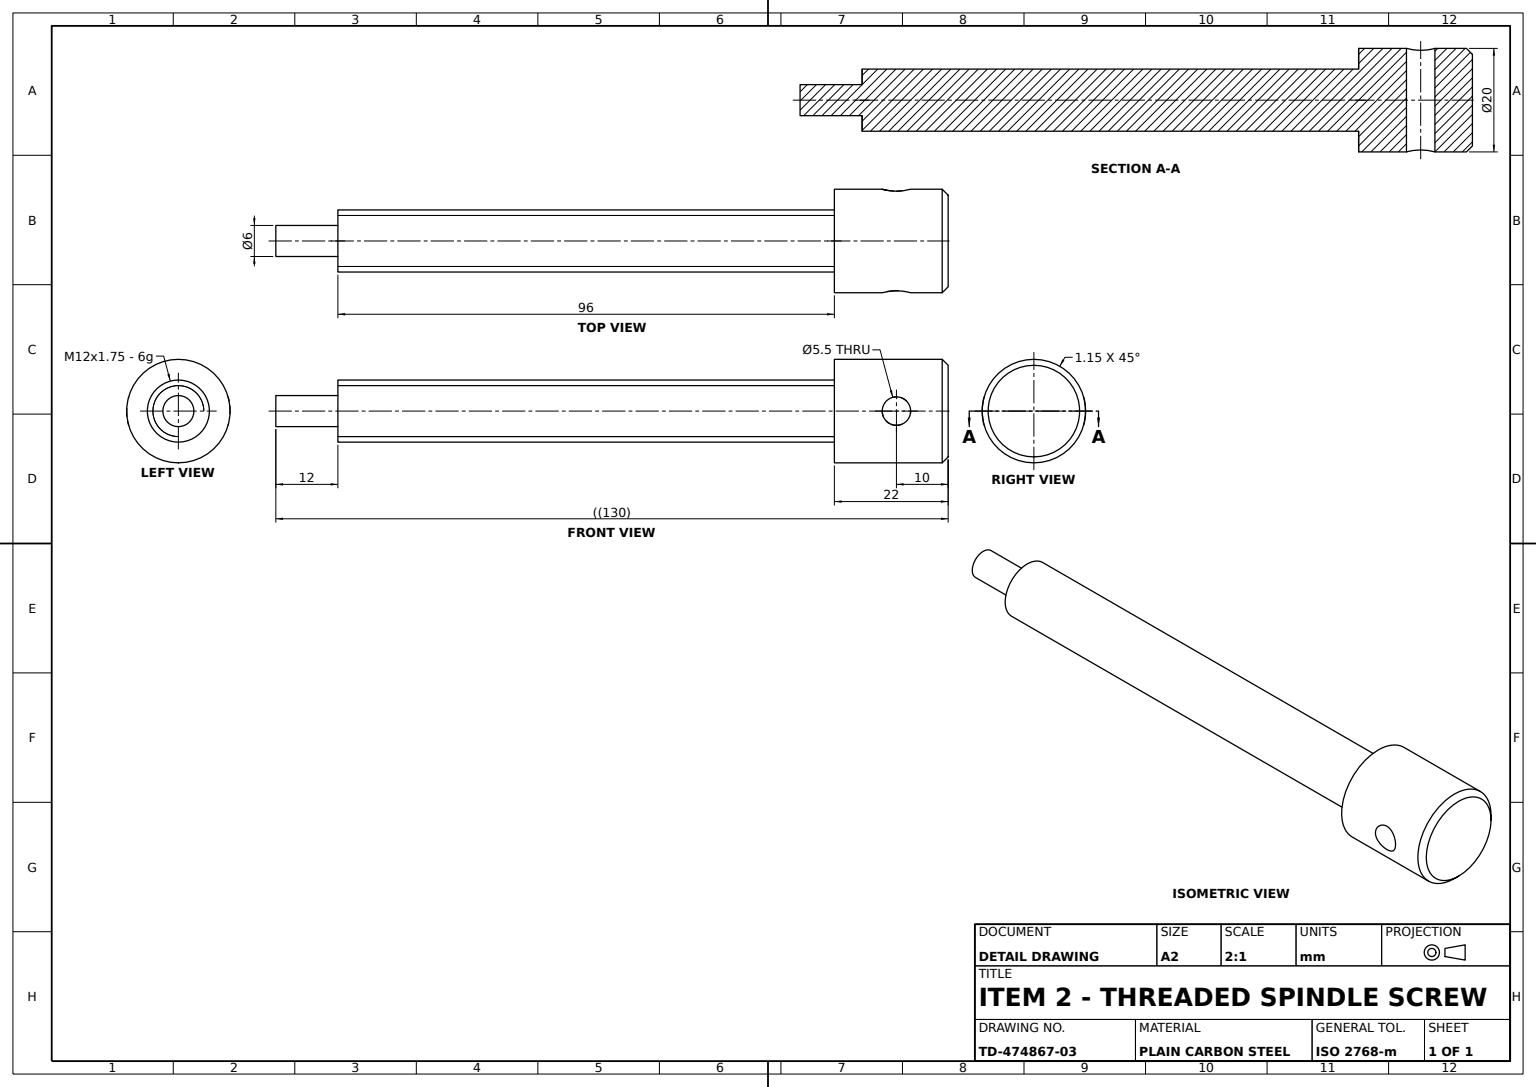
ISO-10303-21;
HEADER;
FILE_DESCRIPTION((''),'2;1');
FILE_NAME('','',(''),(''),'','','');
FILE_SCHEMA(('AUTOMOTIVE_DESIGN'));
ENDSEC;
DATA;
#1=APPLICATION_CONTEXT('');
#2=PRODUCT_CONTEXT('',#1,'mechanical');
#3=PRODUCT('','','',(#2));
#4=PRODUCT_DEFINITION_FORMATION('','',#3);
#5=PRODUCT_DEFINITION_CONTEXT('',#1,'design');
#6=PRODUCT_DEFINITION('','',#4,#5);
#7=PRODUCT_DEFINITION_SHAPE('','',#6);
#8=(LENGTH_UNIT()NAMED_UNIT(*)SI_UNIT(.MILLI.,.METRE.));
#9=(NAMED_UNIT(*)PLANE_ANGLE_UNIT()SI_UNIT($,.RADIAN.));
#10=(NAMED_UNIT(*)SI_UNIT($,.STERADIAN.)SOLID_ANGLE_UNIT());
#11=UNCERTAINTY_MEASURE_WITH_UNIT(LENGTH_MEASURE(1.E-05),#8,'distance_accuracy_value','');
#12=(GEOMETRIC_REPRESENTATION_CONTEXT(3)GLOBAL_UNCERTAINTY_ASSIGNED_CONTEXT((#11))GLOBAL_UNIT_ASSIGNED_CONTEXT((#8,#9,#10))REPRESENTATION_CONTEXT('',''));
#13=CARTESIAN_POINT('',(6.,0.,0.));
#14=VERTEX_POINT('',#13);
#15=CARTESIAN_POINT('',(-6.,0.,0.));
#16=VERTEX_POINT('',#15);
#17=CARTESIAN_POINT('',(0.,0.,0.));
#18=DIRECTION('',(0.,0.,-1.));
#19=DIRECTION('',(-1.,0.,0.));
#20=AXIS2_PLACEMENT_3D('',#17,#18,#19);
#21=CIRCLE('',#20,6.);
#22=EDGE_CURVE('',#14,#16,#21,.T.);
#23=ORIENTED_EDGE('',*,*,#22,.T.);
#24=CARTESIAN_POINT('',(-6.,0.,-96.));
#25=VERTEX_POINT('',#24);
#26=DIRECTION('',(0.,0.,1.));
#27=VECTOR('',#26,1000.);
#28=LINE('',#24,#27);
#29=EDGE_CURVE('',#25,#16,#28,.T.);
#30=ORIENTED_EDGE('',*,*,#29,.F.);
#31=CARTESIAN_POINT('',(6.,0.,-96.));
#32=VERTEX_POINT('',#31);
#33=CARTESIAN_POINT('',(0.,0.,-96.));
#34=AXIS2_PLACEMENT_3D('',#33,#18,#19);
#35=CIRCLE('',#34,6.);
#36=EDGE_CURVE('',#32,#25,#35,.T.);
#37=ORIENTED_EDGE('',*,*,#36,.F.);
#38=LINE('',#31,#27);
#39=EDGE_CURVE('',#32,#14,#38,.T.);
#40=ORIENTED_EDGE('',*,*,#39,.T.);
#41=EDGE_LOOP('',(#23,#30,#37,#40));
#42=FACE_OUTER_BOUND('',#41,.T.);
#43=DIRECTION('',(1.,0.,0.));
#44=AXIS2_PLACEMENT_3D('',#33,#26,#43);
#45=CYLINDRICAL_SURFACE('',#44,6.);
#46=ADVANCED_FACE('',(#42),#45,.T.);
#47=EDGE_CURVE('',#25,#32,#35,.T.);
#48=ORIENTED_EDGE('',*,*,#47,.F.);
#49=ORIENTED_EDGE('',*,*,#29,.T.);
#50=EDGE_CURVE('',#16,#14,#21,.T.);
#51=ORIENTED_EDGE('',*,*,#50,.T.);
#52=ORIENTED_EDGE('',*,*,#39,.F.);
#53=EDGE_LOOP('',(#48,#49,#51,#52));
#54=FACE_OUTER_BOUND('',#53,.T.);
#55=ADVANCED_FACE('',(#54),#45,.T.);
#56=CARTESIAN_POINT('',(0.,-10.,14.75));
#57=VERTEX_POINT('',#56);
#58=CARTESIAN_POINT('',(0.,10.,14.75));
#59=VERTEX_POINT('',#58);
#60=CARTESIAN_POINT('',(0.,-12.,14.75));
#61=DIRECTION('',(0.,1.,0.));
#62=VECTOR('',#61,1000.);
#63=LINE('',#60,#62);
#64=EDGE_CURVE('',#57,#59,#63,.T.);
#65=ORIENTED_EDGE('',*,*,#64,.T.);
#66=CARTESIAN_POINT('',(0.,10.,9.25));
#67=VERTEX_POINT('',#66);
#68=CARTESIAN_POINT('',(0.359941,10.,9.25));
#69=CARTESIAN_POINT('',(0.723396,9.979365,9.322701));
#70=CARTESIAN_POINT('',(1.220421,9.926648,9.529118));
#71=CARTESIAN_POINT('',(1.381339,9.905283,9.61535));
#72=CARTESIAN_POINT('',(1.679306,9.859141,9.814918));
#73=CARTESIAN_POINT('',(1.817154,9.834362,9.928138));
#74=CARTESIAN_POINT('',(2.07085,9.784084,10.181693));
#75=CARTESIAN_POINT('',(2.186063,9.758664,10.322058));
#76=CARTESIAN_POINT('',(2.384629,9.712051,10.618731));
#77=CARTESIAN_POINT('',(2.469436,9.690566,10.776356));
#78=CARTESIAN_POINT('',(2.608794,9.653983,11.111398));
#79=CARTESIAN_POINT('',(2.661177,9.639475,11.283841));
#80=CARTESIAN_POINT('',(2.731712,9.619724,11.635999));
#81=CARTESIAN_POINT('',(2.749963,9.614453,11.818134));
#82=CARTESIAN_POINT('',(2.750036,9.614432,12.180758));
#83=CARTESIAN_POINT('',(2.732315,9.619552,12.35982));
#84=CARTESIAN_POINT('',(2.661932,9.639266,12.713538));
#85=CARTESIAN_POINT('',(2.608512,9.654052,12.889024));
#86=CARTESIAN_POINT('',(2.402035,9.708269,13.386193));
#87=CARTESIAN_POINT('',(2.197588,9.758926,13.691246));
#88=CARTESIAN_POINT('',(1.819481,9.833921,14.069732));
#89=CARTESIAN_POINT('',(1.679617,9.859095,14.184889));
#90=CARTESIAN_POINT('',(1.380712,9.905378,14.385055));
#91=CARTESIAN_POINT('',(1.223196,9.926305,14.469511));
#92=CARTESIAN_POINT('',(0.891943,9.961535,14.607514));
#93=CARTESIAN_POINT('',(0.71648,9.975875,14.661157));
#94=CARTESIAN_POINT('',(0.3624,9.995004,14.731989));
#95=CARTESIAN_POINT('',(0.182598,10.,14.75));
#96=B_SPLINE_CURVE_WITH_KNOTS('',3,(#66,#68,#69,#70,#71,#72,#73,#74,#75,#76,#77,#78,#79,#80,#81,#82,#83,#84,#85,#86,#87,#88,#89,#90,#91,#92,#93,#94,#95,#58),.UNSPECIFIED.,.F.,.F.,(4,2,2,2,2,2,2,2,2,2,2,2,2,2,4),(0.008639567,0.00971922,0.010259046,0.010798872,0.011338698,0.011878525,0.012418351,0.012958177,0.013498004,0.01403783,0.015117482,0.015657309,0.016197135,0.016736961,0.017276787),.UNSPECIFIED.);
#97=EDGE_CURVE('',#67,#59,#96,.T.);
#98=ORIENTED_EDGE('',*,*,#97,.F.);
#99=CARTESIAN_POINT('',(0.,-10.,9.25));
#100=VERTEX_POINT('',#99);
#101=CARTESIAN_POINT('',(0.,-12.,9.25));
#102=LINE('',#101,#62);
#103=EDGE_CURVE('',#100,#67,#102,.T.);
#104=ORIENTED_EDGE('',*,*,#103,.F.);
#105=CARTESIAN_POINT('',(0.182647,-10.,14.75));
#106=CARTESIAN_POINT('',(0.362071,-9.995004,14.731986));
#107=CARTESIAN_POINT('',(0.714787,-9.975985,14.661564));
#108=CARTESIAN_POINT('',(0.889955,-9.961725,14.608244));
#109=CARTESIAN_POINT('',(1.222628,-9.926387,14.469846));
#110=CARTESIAN_POINT('',(1.380263,-9.905435,14.385284));
#111=CARTESIAN_POINT('',(1.678558,-9.859271,14.185669));
#112=CARTESIAN_POINT('',(1.81906,-9.834,14.070113));
#113=CARTESIAN_POINT('',(2.197482,-9.758956,13.691435));
#114=CARTESIAN_POINT('',(2.401961,-9.708283,13.386081));
#115=CARTESIAN_POINT('',(2.608057,-9.654175,12.890267));
#116=CARTESIAN_POINT('',(2.661329,-9.639434,12.716009));
#117=CARTESIAN_POINT('',(2.732273,-9.619566,12.360587));
#118=CARTESIAN_POINT('',(2.749921,-9.614465,12.181551));
#119=CARTESIAN_POINT('',(2.750079,-9.61442,11.820853));
#120=CARTESIAN_POINT('',(2.731967,-9.619652,11.637604));
#121=CARTESIAN_POINT('',(2.661308,-9.639439,11.284169));
#122=CARTESIAN_POINT('',(2.609061,-9.653908,11.112299));
#123=CARTESIAN_POINT('',(2.400961,-9.708551,10.611214));
#124=CARTESIAN_POINT('',(2.198381,-9.75881,10.309153));
#125=CARTESIAN_POINT('',(1.816818,-9.834429,9.927801));
#126=CARTESIAN_POINT('',(1.678899,-9.859205,9.814641));
#127=CARTESIAN_POINT('',(1.381662,-9.905232,9.61557));
#128=CARTESIAN_POINT('',(1.220541,-9.926636,9.529162));
#129=CARTESIAN_POINT('',(0.888778,-9.961822,9.391392));
#130=CARTESIAN_POINT('',(0.717255,-9.975825,9.339031));
#131=CARTESIAN_POINT('',(0.362571,-9.995003,9.268013));
#132=CARTESIAN_POINT('',(0.18002,-10.,9.25));
#133=B_SPLINE_CURVE_WITH_KNOTS('',3,(#56,#105,#106,#107,#108,#109,#110,#111,#112,#113,#114,#115,#116,#117,#118,#119,#120,#121,#122,#123,#124,#125,#126,#127,#128,#129,#130,#131,#132,#99),.UNSPECIFIED.,.F.,.F.,(4,2,2,2,2,2,2,2,2,2,2,2,2,2,4),(0.,0.000539973,0.001079946,0.001619919,0.002159892,0.003239838,0.003779811,0.004319784,0.004859757,0.005399729,0.006479675,0.007019648,0.007559621,0.008099594,0.008639567),.UNSPECIFIED.);
#134=EDGE_CURVE('',#57,#100,#133,.T.);
#135=ORIENTED_EDGE('',*,*,#134,.F.);
#136=EDGE_LOOP('',(#65,#98,#104,#135));
#137=FACE_OUTER_BOUND('',#136,.T.);
#138=CARTESIAN_POINT('',(0.,-12.,12.));
#139=AXIS2_PLACEMENT_3D('',#138,#61,#26);
#140=CYLINDRICAL_SURFACE('',#139,2.75);
#141=ADVANCED_FACE('',(#137),#140,.F.);
#142=CARTESIAN_POINT('',(-0.359941,-10.,9.25));
#143=CARTESIAN_POINT('',(-0.723396,-9.979365,9.322701));
#144=CARTESIAN_POINT('',(-1.220421,-9.926648,9.529118));
#145=CARTESIAN_POINT('',(-1.381339,-9.905283,9.61535));
#146=CARTESIAN_POINT('',(-1.679306,-9.859141,9.814918));
#147=CARTESIAN_POINT('',(-1.817154,-9.834362,9.928138));
#148=CARTESIAN_POINT('',(-2.07085,-9.784084,10.181693));
#149=CARTESIAN_POINT('',(-2.186063,-9.758664,10.322058));
#150=CARTESIAN_POINT('',(-2.384629,-9.712051,10.618731));
#151=CARTESIAN_POINT('',(-2.469436,-9.690566,10.776356));
#152=CARTESIAN_POINT('',(-2.608794,-9.653983,11.111398));
#153=CARTESIAN_POINT('',(-2.661177,-9.639475,11.283841));
#154=CARTESIAN_POINT('',(-2.731712,-9.619724,11.635999));
#155=CARTESIAN_POINT('',(-2.749963,-9.614453,11.818134));
#156=CARTESIAN_POINT('',(-2.750036,-9.614432,12.180758));
#157=CARTESIAN_POINT('',(-2.732315,-9.619552,12.35982));
#158=CARTESIAN_POINT('',(-2.661932,-9.639266,12.713538));
#159=CARTESIAN_POINT('',(-2.608512,-9.654052,12.889024));
#160=CARTESIAN_POINT('',(-2.402035,-9.708269,13.386193));
#161=CARTESIAN_POINT('',(-2.197588,-9.758926,13.691246));
#162=CARTESIAN_POINT('',(-1.819481,-9.833921,14.069732));
#163=CARTESIAN_POINT('',(-1.679617,-9.859095,14.184889));
#164=CARTESIAN_POINT('',(-1.380712,-9.905378,14.385055));
#165=CARTESIAN_POINT('',(-1.223196,-9.926305,14.469511));
#166=CARTESIAN_POINT('',(-0.891943,-9.961535,14.607514));
#167=CARTESIAN_POINT('',(-0.71648,-9.975875,14.661157));
#168=CARTESIAN_POINT('',(-0.3624,-9.995004,14.731989));
#169=CARTESIAN_POINT('',(-0.182598,-10.,14.75));
#170=B_SPLINE_CURVE_WITH_KNOTS('',3,(#99,#142,#143,#144,#145,#146,#147,#148,#149,#150,#151,#152,#153,#154,#155,#156,#157,#158,#159,#160,#161,#162,#163,#164,#165,#166,#167,#168,#169,#56),.UNSPECIFIED.,.F.,.F.,(4,2,2,2,2,2,2,2,2,2,2,2,2,2,4),(0.008639567,0.00971922,0.010259046,0.010798872,0.011338698,0.011878525,0.012418351,0.012958177,0.013498004,0.01403783,0.015117482,0.015657309,0.016197135,0.016736961,0.017276787),.UNSPECIFIED.);
#171=EDGE_CURVE('',#100,#57,#170,.T.);
#172=ORIENTED_EDGE('',*,*,#171,.T.);
#173=ORIENTED_EDGE('',*,*,#134,.T.);
#174=EDGE_LOOP('',(#172,#173));
#175=FACE_BOUND('',#174,.T.);
#176=CARTESIAN_POINT('',(10.,0.,20.85));
#177=VERTEX_POINT('',#176);
#178=CARTESIAN_POINT('',(10.,0.,0.));
#179=VERTEX_POINT('',#178);
#180=CARTESIAN_POINT('',(10.,0.,22.));
#181=VECTOR('',#18,1000.);
#182=LINE('',#180,#181);
#183=EDGE_CURVE('',#177,#179,#182,.T.);
#184=ORIENTED_EDGE('',*,*,#183,.F.);
#185=CARTESIAN_POINT('',(-10.,0.,20.85));
#186=VERTEX_POINT('',#185);
#187=CARTESIAN_POINT('',(0.,0.,20.85));
#188=AXIS2_PLACEMENT_3D('',#187,#18,#43);
#189=CIRCLE('',#188,10.);
#190=EDGE_CURVE('',#177,#186,#189,.T.);
#191=ORIENTED_EDGE('',*,*,#190,.T.);
#192=CARTESIAN_POINT('',(-10.,0.,0.));
#193=VERTEX_POINT('',#192);
#194=CARTESIAN_POINT('',(-10.,0.,22.));
#195=LINE('',#194,#181);
#196=EDGE_CURVE('',#186,#193,#195,.T.);
#197=ORIENTED_EDGE('',*,*,#196,.T.);
#198=AXIS2_PLACEMENT_3D('',#17,#26,#43);
#199=CIRCLE('',#198,10.);
#200=EDGE_CURVE('',#193,#179,#199,.T.);
#201=ORIENTED_EDGE('',*,*,#200,.T.);
#202=EDGE_LOOP('',(#184,#191,#197,#201));
#203=FACE_OUTER_BOUND('',#202,.T.);
#204=CARTESIAN_POINT('',(0.,0.,22.));
#205=AXIS2_PLACEMENT_3D('',#204,#18,#19);
#206=CYLINDRICAL_SURFACE('',#205,10.);
#207=ADVANCED_FACE('',(#175,#203),#206,.T.);
#208=ORIENTED_EDGE('',*,*,#36,.T.);
#209=ORIENTED_EDGE('',*,*,#47,.T.);
#210=EDGE_LOOP('',(#208,#209));
#211=FACE_OUTER_BOUND('',#210,.T.);
#212=CARTESIAN_POINT('',(3.,0.,-96.));
#213=VERTEX_POINT('',#212);
#214=CARTESIAN_POINT('',(-3.,0.,-96.));
#215=VERTEX_POINT('',#214);
#216=CIRCLE('',#34,3.);
#217=EDGE_CURVE('',#213,#215,#216,.T.);
#218=ORIENTED_EDGE('',*,*,#217,.F.);
#219=EDGE_CURVE('',#215,#213,#216,.T.);
#220=ORIENTED_EDGE('',*,*,#219,.F.);
#221=EDGE_LOOP('',(#218,#220));
#222=FACE_BOUND('',#221,.T.);
#223=PLANE('',#34);
#224=ADVANCED_FACE('',(#211,#222),#223,.T.);
#225=ORIENTED_EDGE('',*,*,#97,.T.);
#226=CARTESIAN_POINT('',(-0.182647,10.,14.75));
#227=CARTESIAN_POINT('',(-0.362071,9.995004,14.731986));
#228=CARTESIAN_POINT('',(-0.714787,9.975985,14.661564));
#229=CARTESIAN_POINT('',(-0.889955,9.961725,14.608244));
#230=CARTESIAN_POINT('',(-1.222628,9.926387,14.469846));
#231=CARTESIAN_POINT('',(-1.380263,9.905435,14.385284));
#232=CARTESIAN_POINT('',(-1.678558,9.859271,14.185669));
#233=CARTESIAN_POINT('',(-1.81906,9.834,14.070113));
#234=CARTESIAN_POINT('',(-2.197482,9.758956,13.691435));
#235=CARTESIAN_POINT('',(-2.401961,9.708283,13.386081));
#236=CARTESIAN_POINT('',(-2.608057,9.654175,12.890267));
#237=CARTESIAN_POINT('',(-2.661329,9.639434,12.716009));
#238=CARTESIAN_POINT('',(-2.732273,9.619566,12.360587));
#239=CARTESIAN_POINT('',(-2.749921,9.614465,12.181551));
#240=CARTESIAN_POINT('',(-2.750079,9.61442,11.820853));
#241=CARTESIAN_POINT('',(-2.731967,9.619652,11.637604));
#242=CARTESIAN_POINT('',(-2.661308,9.639439,11.284169));
#243=CARTESIAN_POINT('',(-2.609061,9.653908,11.112299));
#244=CARTESIAN_POINT('',(-2.400961,9.708551,10.611214));
#245=CARTESIAN_POINT('',(-2.198381,9.75881,10.309153));
#246=CARTESIAN_POINT('',(-1.816818,9.834429,9.927801));
#247=CARTESIAN_POINT('',(-1.678899,9.859205,9.814641));
#248=CARTESIAN_POINT('',(-1.381662,9.905232,9.61557));
#249=CARTESIAN_POINT('',(-1.220541,9.926636,9.529162));
#250=CARTESIAN_POINT('',(-0.888778,9.961822,9.391392));
#251=CARTESIAN_POINT('',(-0.717255,9.975825,9.339031));
#252=CARTESIAN_POINT('',(-0.362571,9.995003,9.268013));
#253=CARTESIAN_POINT('',(-0.18002,10.,9.25));
#254=B_SPLINE_CURVE_WITH_KNOTS('',3,(#58,#226,#227,#228,#229,#230,#231,#232,#233,#234,#235,#236,#237,#238,#239,#240,#241,#242,#243,#244,#245,#246,#247,#248,#249,#250,#251,#252,#253,#66),.UNSPECIFIED.,.F.,.F.,(4,2,2,2,2,2,2,2,2,2,2,2,2,2,4),(0.,0.000539973,0.001079946,0.001619919,0.002159892,0.003239838,0.003779811,0.004319784,0.004859757,0.005399729,0.006479675,0.007019648,0.007559621,0.008099594,0.008639567),.UNSPECIFIED.);
#255=EDGE_CURVE('',#59,#67,#254,.T.);
#256=ORIENTED_EDGE('',*,*,#255,.T.);
#257=EDGE_LOOP('',(#225,#256));
#258=FACE_BOUND('',#257,.T.);
#259=ORIENTED_EDGE('',*,*,#183,.T.);
#260=EDGE_CURVE('',#179,#193,#199,.T.);
#261=ORIENTED_EDGE('',*,*,#260,.T.);
#262=ORIENTED_EDGE('',*,*,#196,.F.);
#263=EDGE_CURVE('',#186,#177,#189,.T.);
#264=ORIENTED_EDGE('',*,*,#263,.T.);
#265=EDGE_LOOP('',(#259,#261,#262,#264));
#266=FACE_OUTER_BOUND('',#265,.T.);
#267=ADVANCED_FACE('',(#258,#266),#206,.T.);
#268=ORIENTED_EDGE('',*,*,#103,.T.);
#269=ORIENTED_EDGE('',*,*,#255,.F.);
#270=ORIENTED_EDGE('',*,*,#64,.F.);
#271=ORIENTED_EDGE('',*,*,#171,.F.);
#272=EDGE_LOOP('',(#268,#269,#270,#271));
#273=FACE_OUTER_BOUND('',#272,.T.);
#274=ADVANCED_FACE('',(#273),#140,.F.);
#275=ORIENTED_EDGE('',*,*,#22,.F.);
#276=ORIENTED_EDGE('',*,*,#50,.F.);
#277=EDGE_LOOP('',(#275,#276));
#278=FACE_BOUND('',#277,.T.);
#279=ORIENTED_EDGE('',*,*,#200,.F.);
#280=ORIENTED_EDGE('',*,*,#260,.F.);
#281=EDGE_LOOP('',(#279,#280));
#282=FACE_OUTER_BOUND('',#281,.T.);
#283=PLANE('',#198);
#284=ADVANCED_FACE('',(#278,#282),#283,.F.);
#285=CARTESIAN_POINT('',(-8.85,0.,22.));
#286=VERTEX_POINT('',#285);
#287=CARTESIAN_POINT('',(8.85,0.,22.));
#288=VERTEX_POINT('',#287);
#289=AXIS2_PLACEMENT_3D('',#204,#26,#43);
#290=CIRCLE('',#289,8.85);
#291=EDGE_CURVE('',#286,#288,#290,.T.);
#292=ORIENTED_EDGE('',*,*,#291,.T.);
#293=EDGE_CURVE('',#288,#286,#290,.T.);
#294=ORIENTED_EDGE('',*,*,#293,.T.);
#295=EDGE_LOOP('',(#292,#294));
#296=FACE_OUTER_BOUND('',#295,.T.);
#297=PLANE('',#289);
#298=ADVANCED_FACE('',(#296),#297,.T.);
#299=CARTESIAN_POINT('',(-3.,0.,-108.));
#300=VERTEX_POINT('',#299);
#301=CARTESIAN_POINT('',(3.,0.,-108.));
#302=VERTEX_POINT('',#301);
#303=CARTESIAN_POINT('',(0.,0.,-108.));
#304=AXIS2_PLACEMENT_3D('',#303,#18,#19);
#305=CIRCLE('',#304,3.);
#306=EDGE_CURVE('',#300,#302,#305,.T.);
#307=ORIENTED_EDGE('',*,*,#306,.F.);
#308=LINE('',#299,#27);
#309=EDGE_CURVE('',#300,#215,#308,.T.);
#310=ORIENTED_EDGE('',*,*,#309,.T.);
#311=ORIENTED_EDGE('',*,*,#219,.T.);
#312=LINE('',#301,#27);
#313=EDGE_CURVE('',#302,#213,#312,.T.);
#314=ORIENTED_EDGE('',*,*,#313,.F.);
#315=EDGE_LOOP('',(#307,#310,#311,#314));
#316=FACE_OUTER_BOUND('',#315,.T.);
#317=AXIS2_PLACEMENT_3D('',#303,#26,#43);
#318=CYLINDRICAL_SURFACE('',#317,3.);
#319=ADVANCED_FACE('',(#316),#318,.T.);
#320=ORIENTED_EDGE('',*,*,#263,.F.);
#321=DIRECTION('',(-0.707106781,0.,-0.707106781));
#322=VECTOR('',#321,1000.);
#323=LINE('',#285,#322);
#324=EDGE_CURVE('',#286,#186,#323,.T.);
#325=ORIENTED_EDGE('',*,*,#324,.F.);
#326=ORIENTED_EDGE('',*,*,#293,.F.);
#327=DIRECTION('',(0.707106781,0.,-0.707106781));
#328=VECTOR('',#327,1000.);
#329=LINE('',#287,#328);
#330=EDGE_CURVE('',#288,#177,#329,.T.);
#331=ORIENTED_EDGE('',*,*,#330,.T.);
#332=EDGE_LOOP('',(#320,#325,#326,#331));
#333=FACE_OUTER_BOUND('',#332,.T.);
#334=CONICAL_SURFACE('',#205,8.85,0.785398163);
#335=ADVANCED_FACE('',(#333),#334,.T.);
#336=ORIENTED_EDGE('',*,*,#306,.T.);
#337=EDGE_CURVE('',#302,#300,#305,.T.);
#338=ORIENTED_EDGE('',*,*,#337,.T.);
#339=EDGE_LOOP('',(#336,#338));
#340=FACE_OUTER_BOUND('',#339,.T.);
#341=PLANE('',#304);
#342=ADVANCED_FACE('',(#340),#341,.T.);
#343=ORIENTED_EDGE('',*,*,#309,.F.);
#344=ORIENTED_EDGE('',*,*,#337,.F.);
#345=ORIENTED_EDGE('',*,*,#313,.T.);
#346=ORIENTED_EDGE('',*,*,#217,.T.);
#347=EDGE_LOOP('',(#343,#344,#345,#346));
#348=FACE_OUTER_BOUND('',#347,.T.);
#349=ADVANCED_FACE('',(#348),#318,.T.);
#350=ORIENTED_EDGE('',*,*,#190,.F.);
#351=ORIENTED_EDGE('',*,*,#330,.F.);
#352=ORIENTED_EDGE('',*,*,#291,.F.);
#353=ORIENTED_EDGE('',*,*,#324,.T.);
#354=EDGE_LOOP('',(#350,#351,#352,#353));
#355=FACE_OUTER_BOUND('',#354,.T.);
#356=ADVANCED_FACE('',(#355),#334,.T.);
#357=CLOSED_SHELL('',(#46,#55,#141,#207,#224,#267,#274,#284,#298,#319,#335,#342,#349,#356));
#358=MANIFOLD_SOLID_BREP('',#357);
#359=ADVANCED_BREP_SHAPE_REPRESENTATION('',(#358),#12);
#360=SHAPE_DEFINITION_REPRESENTATION(#7,#359);
ENDSEC;
END-ISO-10303-21;
